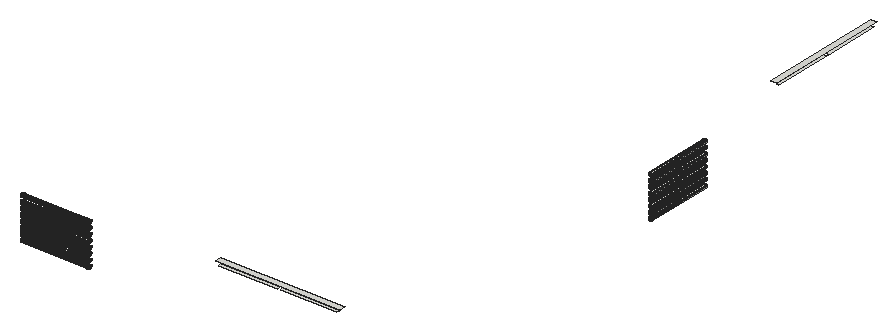
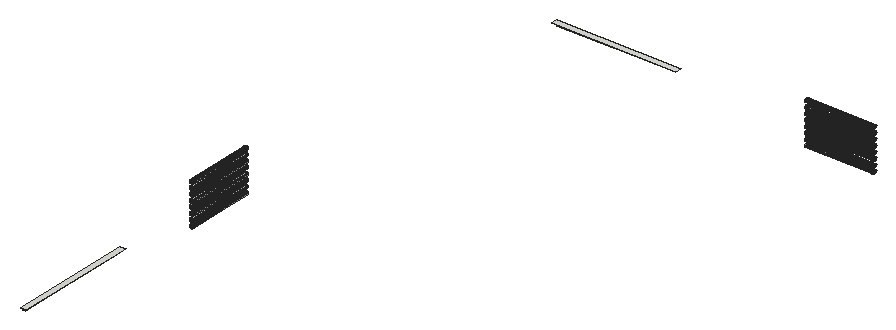
# SketchUp Ruby script. Lengths in inches.
U = 1.inch
M = Sketchup.active_model
def pt(a) = Geom::Point3d.new(a.map { |v| v * U })
def face(e, loops, mat)
  f = e.add_face(loops[0].map { |a| pt(a) })
  loops[1..].each { |l| e.add_face(l.map { |a| pt(a) }).erase! }
  f.material = f.back_material = mat if mat
  f
end
# faces: each face lists its corners as indices into pts; further lists are holes
def faces(e, pts, list, mat = nil) = list.each { |f| face(e, (f[0].is_a?(Array) ? f : [f]).map { |l| l.map { |i| pts[i] } }, mat) }
# xy, xz, yz: faces in a plane at the given z, y or x. An outline is a flat list of corners, or four numbers for a rectangle; further outlines are holes
def ring(l) = l.size == 4 ? [[l[0], l[1]], [l[2], l[1]], [l[2], l[3]], [l[0], l[3]]] : l.each_slice(2).to_a
def flat(e, list, mat, &to3) = list.each { |f| face(e, (f[0].is_a?(Array) ? f : [f]).map { |l| ring(l).map { |u, v| to3.(u, v) } }, mat) }
def xy(e, z, list, mat = nil) = flat(e, list, mat) { |x, y| [x, y, z] }
def xz(e, y, list, mat = nil) = flat(e, list, mat) { |x, z| [x, y, z] }
def yz(e, x, list, mat = nil) = flat(e, list, mat) { |y, z| [x, y, z] }
def lines(e, pts, list) = list.each { |a, b| e.add_line(pt(pts[a]), pt(pts[b])) }
# prism: a flat outline (further loops are holes) pulled along v
def prism(e, loops, v, mat = nil)
  f = face(e, loops, mat); d = Geom::Vector3d.new(v.map { |x| x * U })
  f.pushpull(f.normal.samedirection?(d) ? d.length : -d.length)
end
def box(e, o, s, mat = nil) = prism(e, [[o, [o[0] + s[0], o[1], o[2]], [o[0] + s[0], o[1] + s[1], o[2]], [o[0], o[1] + s[1], o[2]]]], [0, 0, s[2]], mat)
def at(x, y, z, deg = 0) = Geom::Transformation.translation(pt([x, y, z])) * Geom::Transformation.rotation(ORIGIN, Z_AXIS, deg.degrees)
def axes(o, x, y, z) = Geom::Transformation.new([*x, 0, *y, 0, *z, 0, *pt(o).to_a, 1])
def part(name) = M.definitions.add(name)
# library, detail: a bought-in or finely detailed component or shape, given as its bounding box
def library(name, o, s) = part(name).tap { |d| box(d.entities, o, s) }
def detail(e, o, s) = box(e.add_group.entities, o, s)
def put(e, d, t, mat = nil) = e.add_instance(d, t).tap { |i| i.material = mat if mat }
def group(e, t, mat = nil) = e.add_group.tap { |g| g.transformation = t; g.material = mat if mat }.entities
root = M.entities
xy(root,1007.61,[[1161.2,84.8125,1285.04,90.8125],[1291.04,84.8125,1408.89,90.8125],[1494,1126.01,1500,1249.86],[1494,1255.86,1500,1373.7]])
xy(root,1013.61,[[1155.2,84.8125,1414.89,96.8125],[1488,1120.01,1500,1379.7]])
p = [[922.01,48.34,933.02],[922.01,47.38,933.14],[778.64,47.38,933.14],[778.64,48.34,933.02],[922.01,49.29,933.14],[778.64,49.29,933.14],
  [1535.52,886.83,933.14],[1536.47,886.83,933.02],[1536.47,743.45,933.02],[1535.52,743.45,933.14],[1537.43,886.83,933.14],[1537.43,743.45,933.14],
  [922.01,46.5,933.51],[778.64,46.5,933.51],[922.01,50.18,933.51],[778.64,50.18,933.51],[1534.63,886.83,933.51],[1534.63,743.45,933.51],
  [1538.32,886.83,933.51],[1538.32,743.45,933.51],[922.01,45.73,934.1],[778.64,45.73,934.1],[922.01,50.95,934.1],[778.64,50.95,934.1],
  [1533.87,886.83,934.1],[1533.87,743.45,934.1],[1539.08,886.83,934.1],[1539.08,743.45,934.1],[922.01,45.15,934.86],[778.64,45.15,934.86],
  [922.01,51.53,934.86],[778.64,51.53,934.86],[1533.28,886.83,934.86],[1533.28,743.45,934.86],[1539.67,886.83,934.86],[1539.67,743.45,934.86],
  [922.01,44.78,935.75],[778.64,44.78,935.75],[922.01,51.9,935.75],[778.64,51.9,935.75],[1532.91,886.83,935.75],[1532.91,743.45,935.75],
  [1540.03,886.83,935.75],[1540.03,743.45,935.75],[922.01,44.65,936.7],[778.64,44.65,936.7],[922.01,52.03,936.7],[778.64,52.03,936.7],
  [1532.79,886.83,936.7],[1532.79,743.45,936.7],[1540.16,886.83,936.7],[1540.16,743.45,936.7],[922.01,44.78,937.66],[778.64,44.78,937.66],
  [922.01,51.9,937.66],[778.64,51.9,937.66],[1532.91,886.83,937.66],[1532.91,743.45,937.66],[1540.03,886.83,937.66],[1540.03,743.45,937.66],
  [922.01,45.15,938.55],[778.64,45.15,938.55],[922.01,51.53,938.55],[778.64,51.53,938.55],[1533.28,886.83,938.55],[1533.28,743.45,938.55],
  [1539.67,886.83,938.55],[1539.67,743.45,938.55],[922.01,45.73,939.3125],[778.64,45.73,939.3125],[922.01,50.95,939.3125],[778.64,50.95,939.3125],
  [1533.87,886.83,939.3125],[1533.87,743.45,939.3125],[1539.08,886.83,939.3125],[1539.08,743.45,939.3125],[922.01,46.5,939.9],[778.64,46.5,939.9],
  [922.01,50.18,939.9],[778.64,50.18,939.9],[1534.63,886.83,939.9],[1534.63,743.45,939.9],[1538.32,886.83,939.9],[1538.32,743.45,939.9],
  [922.01,47.38,940.27],[778.64,47.38,940.27],[922.01,49.29,940.27],[778.64,49.29,940.27],[1535.52,886.83,940.27],[1535.52,743.45,940.27],
  [1537.43,886.83,940.27],[1537.43,743.45,940.27],[922.01,48.34,940.39],[778.64,48.34,940.39],[1536.47,886.83,940.39],[1536.47,743.45,940.39],
  [922.01,48.34,945.02],[922.01,47.38,945.14],[778.64,47.38,945.14],[778.64,48.34,945.02],[922.01,49.29,945.14],[778.64,49.29,945.14],
  [1535.52,886.83,945.14],[1536.47,886.83,945.02],[1536.47,743.45,945.02],[1535.52,743.45,945.14],[1537.43,886.83,945.14],[1537.43,743.45,945.14],
  [922.01,46.5,945.51],[778.64,46.5,945.51],[922.01,50.18,945.51],[778.64,50.18,945.51],[1534.63,886.83,945.51],[1534.63,743.45,945.51],
  [1538.32,886.83,945.51],[1538.32,743.45,945.51],[922.01,45.73,946.1],[778.64,45.73,946.1],[922.01,50.95,946.1],[778.64,50.95,946.1],
  [1533.87,886.83,946.1],[1533.87,743.45,946.1],[1539.08,886.83,946.1],[1539.08,743.45,946.1],[922.01,45.15,946.86],[778.64,45.15,946.86],
  [922.01,51.53,946.86],[778.64,51.53,946.86],[1533.28,886.83,946.86],[1533.28,743.45,946.86],[1539.67,886.83,946.86],[1539.67,743.45,946.86],
  [922.01,44.78,947.75],[778.64,44.78,947.75],[922.01,51.9,947.75],[778.64,51.9,947.75],[1532.91,886.83,947.75],[1532.91,743.45,947.75],
  [1540.03,886.83,947.75],[1540.03,743.45,947.75],[922.01,44.65,948.7],[778.64,44.65,948.7],[922.01,52.03,948.7],[778.64,52.03,948.7],
  [1532.79,886.83,948.7],[1532.79,743.45,948.7],[1540.16,886.83,948.7],[1540.16,743.45,948.7],[922.01,44.78,949.66],[778.64,44.78,949.66],
  [922.01,51.9,949.66],[778.64,51.9,949.66],[1532.91,886.83,949.66],[1532.91,743.45,949.66],[1540.03,886.83,949.66],[1540.03,743.45,949.66],
  [922.01,45.15,950.55],[778.64,45.15,950.55],[922.01,51.53,950.55],[778.64,51.53,950.55],[1533.28,886.83,950.55],[1533.28,743.45,950.55],
  [1539.67,886.83,950.55],[1539.67,743.45,950.55],[922.01,45.73,951.3125],[778.64,45.73,951.3125],[922.01,50.95,951.3125],[778.64,50.95,951.3125],
  [1533.87,886.83,951.3125],[1533.87,743.45,951.3125],[1539.08,886.83,951.3125],[1539.08,743.45,951.3125],[922.01,46.5,951.9],[778.64,46.5,951.9],
  [922.01,50.18,951.9],[778.64,50.18,951.9],[1534.63,886.83,951.9],[1534.63,743.45,951.9],[1538.32,886.83,951.9],[1538.32,743.45,951.9],
  [922.01,47.38,952.27],[778.64,47.38,952.27],[922.01,49.29,952.27],[778.64,49.29,952.27],[1535.52,886.83,952.27],[1535.52,743.45,952.27],
  [1537.43,886.83,952.27],[1537.43,743.45,952.27],[922.01,48.34,952.39],[778.64,48.34,952.39],[1536.47,886.83,952.39],[1536.47,743.45,952.39],
  [922.01,48.34,957.02],[922.01,47.38,957.14],[778.64,47.38,957.14],[778.64,48.34,957.02],[922.01,49.29,957.14],[778.64,49.29,957.14],
  [1535.52,886.83,957.14],[1536.47,886.83,957.02],[1536.47,743.45,957.02],[1535.52,743.45,957.14],[1537.43,886.83,957.14],[1537.43,743.45,957.14],
  [922.01,46.5,957.51],[778.64,46.5,957.51],[922.01,50.18,957.51],[778.64,50.18,957.51],[1534.63,886.83,957.51],[1534.63,743.45,957.51],
  [1538.32,886.83,957.51],[1538.32,743.45,957.51],[922.01,45.73,958.1],[778.64,45.73,958.1],[922.01,50.95,958.1],[778.64,50.95,958.1],
  [1533.87,886.83,958.1],[1533.87,743.45,958.1],[1539.08,886.83,958.1],[1539.08,743.45,958.1],[922.01,45.15,958.86],[778.64,45.15,958.86],
  [922.01,51.53,958.86],[778.64,51.53,958.86],[1533.28,886.83,958.86],[1533.28,743.45,958.86],[1539.67,886.83,958.86],[1539.67,743.45,958.86],
  [922.01,44.78,959.75],[778.64,44.78,959.75],[922.01,51.9,959.75],[778.64,51.9,959.75],[1532.91,886.83,959.75],[1532.91,743.45,959.75],
  [1540.03,886.83,959.75],[1540.03,743.45,959.75],[922.01,44.65,960.7],[778.64,44.65,960.7],[922.01,52.03,960.7],[778.64,52.03,960.7],
  [1532.79,886.83,960.7],[1532.79,743.45,960.7],[1540.16,886.83,960.7],[1540.16,743.45,960.7],[922.01,44.78,961.66],[778.64,44.78,961.66],
  [922.01,51.9,961.66],[778.64,51.9,961.66],[1532.91,886.83,961.66],[1532.91,743.45,961.66],[1540.03,886.83,961.66],[1540.03,743.45,961.66],
  [922.01,45.15,962.55],[778.64,45.15,962.55],[922.01,51.53,962.55],[778.64,51.53,962.55],[1533.28,886.83,962.55],[1533.28,743.45,962.55],
  [1539.67,886.83,962.55],[1539.67,743.45,962.55],[922.01,45.73,963.3125],[778.64,45.73,963.3125],[922.01,50.95,963.3125],[778.64,50.95,963.3125],
  [1533.87,886.83,963.3125],[1533.87,743.45,963.3125],[1539.08,886.83,963.3125],[1539.08,743.45,963.3125],[922.01,46.5,963.9],[778.64,46.5,963.9],
  [922.01,50.18,963.9],[778.64,50.18,963.9],[1534.63,886.83,963.9],[1534.63,743.45,963.9],[1538.32,886.83,963.9],[1538.32,743.45,963.9],
  [922.01,47.38,964.27],[778.64,47.38,964.27],[922.01,49.29,964.27],[778.64,49.29,964.27],[1535.52,886.83,964.27],[1535.52,743.45,964.27],
  [1537.43,886.83,964.27],[1537.43,743.45,964.27],[922.01,48.34,964.39],[778.64,48.34,964.39],[1536.47,886.83,964.39],[1536.47,743.45,964.39],
  [922.01,48.34,969.02],[922.01,47.38,969.14],[778.64,47.38,969.14],[778.64,48.34,969.02],[922.01,49.29,969.14],[778.64,49.29,969.14],
  [1535.52,886.83,969.14],[1536.47,886.83,969.02],[1536.47,743.45,969.02],[1535.52,743.45,969.14],[1537.43,886.83,969.14],[1537.43,743.45,969.14],
  [922.01,46.5,969.51],[778.64,46.5,969.51],[922.01,50.18,969.51],[778.64,50.18,969.51],[1534.63,886.83,969.51],[1534.63,743.45,969.51],
  [1538.32,886.83,969.51],[1538.32,743.45,969.51],[922.01,45.73,970.1],[778.64,45.73,970.1],[922.01,50.95,970.1],[778.64,50.95,970.1],
  [1533.87,886.83,970.1],[1533.87,743.45,970.1],[1539.08,886.83,970.1],[1539.08,743.45,970.1],[922.01,45.15,970.86],[778.64,45.15,970.86],
  [922.01,51.53,970.86],[778.64,51.53,970.86],[1533.28,886.83,970.86],[1533.28,743.45,970.86],[1539.67,886.83,970.86],[1539.67,743.45,970.86],
  [922.01,44.78,971.75],[778.64,44.78,971.75],[922.01,51.9,971.75],[778.64,51.9,971.75],[1532.91,886.83,971.75],[1532.91,743.45,971.75],
  [1540.03,886.83,971.75],[1540.03,743.45,971.75],[922.01,44.65,972.7],[778.64,44.65,972.7],[922.01,52.03,972.7],[778.64,52.03,972.7],
  [1532.79,886.83,972.7],[1532.79,743.45,972.7],[1540.16,886.83,972.7],[1540.16,743.45,972.7],[922.01,44.78,973.66],[778.64,44.78,973.66],
  [922.01,51.9,973.66],[778.64,51.9,973.66],[1532.91,886.83,973.66],[1532.91,743.45,973.66],[1540.03,886.83,973.66],[1540.03,743.45,973.66],
  [922.01,45.15,974.55],[778.64,45.15,974.55],[922.01,51.53,974.55],[778.64,51.53,974.55],[1533.28,886.83,974.55],[1533.28,743.45,974.55],
  [1539.67,886.83,974.55],[1539.67,743.45,974.55],[922.01,45.73,975.3125],[778.64,45.73,975.3125],[922.01,50.95,975.3125],[778.64,50.95,975.3125],
  [1533.87,886.83,975.3125],[1533.87,743.45,975.3125],[1539.08,886.83,975.3125],[1539.08,743.45,975.3125],[922.01,46.5,975.9],[778.64,46.5,975.9],
  [922.01,50.18,975.9],[778.64,50.18,975.9],[1534.63,886.83,975.9],[1534.63,743.45,975.9],[1538.32,886.83,975.9],[1538.32,743.45,975.9],
  [922.01,47.38,976.27],[778.64,47.38,976.27],[922.01,49.29,976.27],[778.64,49.29,976.27],[1535.52,886.83,976.27],[1535.52,743.45,976.27],
  [1537.43,886.83,976.27],[1537.43,743.45,976.27],[922.01,48.34,976.39],[778.64,48.34,976.39],[1536.47,886.83,976.39],[1536.47,743.45,976.39],
  [922.01,48.34,981.02],[922.01,47.38,981.14],[778.64,47.38,981.14],[778.64,48.34,981.02],[922.01,49.29,981.14],[778.64,49.29,981.14],
  [1535.52,886.83,981.14],[1536.47,886.83,981.02],[1536.47,743.45,981.02],[1535.52,743.45,981.14],[1537.43,886.83,981.14],[1537.43,743.45,981.14],
  [922.01,46.5,981.51],[778.64,46.5,981.51],[922.01,50.18,981.51],[778.64,50.18,981.51],[1534.63,886.83,981.51],[1534.63,743.45,981.51],
  [1538.32,886.83,981.51],[1538.32,743.45,981.51],[922.01,45.73,982.1],[778.64,45.73,982.1],[922.01,50.95,982.1],[778.64,50.95,982.1],
  [1533.87,886.83,982.1],[1533.87,743.45,982.1],[1539.08,886.83,982.1],[1539.08,743.45,982.1],[922.01,45.15,982.86],[778.64,45.15,982.86],
  [922.01,51.53,982.86],[778.64,51.53,982.86],[1533.28,886.83,982.86],[1533.28,743.45,982.86],[1539.67,886.83,982.86],[1539.67,743.45,982.86],
  [922.01,44.78,983.75],[778.64,44.78,983.75],[922.01,51.9,983.75],[778.64,51.9,983.75],[1532.91,886.83,983.75],[1532.91,743.45,983.75],
  [1540.03,886.83,983.75],[1540.03,743.45,983.75],[922.01,44.65,984.7],[778.64,44.65,984.7],[922.01,52.03,984.7],[778.64,52.03,984.7],
  [1532.79,886.83,984.7],[1532.79,743.45,984.7],[1540.16,886.83,984.7],[1540.16,743.45,984.7],[922.01,44.78,985.66],[778.64,44.78,985.66],
  [922.01,51.9,985.66],[778.64,51.9,985.66],[1532.91,886.83,985.66],[1532.91,743.45,985.66],[1540.03,886.83,985.66],[1540.03,743.45,985.66],
  [922.01,45.15,986.55],[778.64,45.15,986.55],[922.01,51.53,986.55],[778.64,51.53,986.55],[1533.28,886.83,986.55],[1533.28,743.45,986.55],
  [1539.67,886.83,986.55],[1539.67,743.45,986.55],[922.01,45.73,987.3125],[778.64,45.73,987.3125],[922.01,50.95,987.3125],[778.64,50.95,987.3125],
  [1533.87,886.83,987.3125],[1533.87,743.45,987.3125],[1539.08,886.83,987.3125],[1539.08,743.45,987.3125],[922.01,46.5,987.9],[778.64,46.5,987.9],
  [922.01,50.18,987.9],[778.64,50.18,987.9],[1534.63,886.83,987.9],[1534.63,743.45,987.9],[1538.32,886.83,987.9],[1538.32,743.45,987.9],
  [922.01,47.38,988.27],[778.64,47.38,988.27],[922.01,49.29,988.27],[778.64,49.29,988.27],[1535.52,886.83,988.27],[1535.52,743.45,988.27],
  [1537.43,886.83,988.27],[1537.43,743.45,988.27],[922.01,48.34,988.39],[778.64,48.34,988.39],[1536.47,886.83,988.39],[1536.47,743.45,988.39],
  [922.01,48.34,993.02],[922.01,47.38,993.14],[778.64,47.38,993.14],[778.64,48.34,993.02],[922.01,49.29,993.14],[778.64,49.29,993.14],
  [1535.52,886.83,993.14],[1536.47,886.83,993.02],[1536.47,743.45,993.02],[1535.52,743.45,993.14],[1537.43,886.83,993.14],[1537.43,743.45,993.14],
  [922.01,46.5,993.51],[778.64,46.5,993.51],[922.01,50.18,993.51],[778.64,50.18,993.51],[1534.63,886.83,993.51],[1534.63,743.45,993.51],
  [1538.32,886.83,993.51],[1538.32,743.45,993.51],[922.01,45.73,994.1],[778.64,45.73,994.1],[922.01,50.95,994.1],[778.64,50.95,994.1],
  [1533.87,886.83,994.1],[1533.87,743.45,994.1],[1539.08,886.83,994.1],[1539.08,743.45,994.1],[922.01,45.15,994.86],[778.64,45.15,994.86],
  [922.01,51.53,994.86],[778.64,51.53,994.86],[1533.28,886.83,994.86],[1533.28,743.45,994.86],[1539.67,886.83,994.86],[1539.67,743.45,994.86],
  [922.01,44.78,995.75],[778.64,44.78,995.75],[922.01,51.9,995.75],[778.64,51.9,995.75],[1532.91,886.83,995.75],[1532.91,743.45,995.75],
  [1540.03,886.83,995.75],[1540.03,743.45,995.75],[922.01,44.65,996.7],[778.64,44.65,996.7],[922.01,52.03,996.7],[778.64,52.03,996.7],
  [1532.79,886.83,996.7],[1532.79,743.45,996.7],[1540.16,886.83,996.7],[1540.16,743.45,996.7],[922.01,44.78,997.66],[778.64,44.78,997.66],
  [922.01,51.9,997.66],[778.64,51.9,997.66],[1532.91,886.83,997.66],[1532.91,743.45,997.66],[1540.03,886.83,997.66],[1540.03,743.45,997.66],
  [922.01,45.15,998.55],[778.64,45.15,998.55],[922.01,51.53,998.55],[778.64,51.53,998.55],[1533.28,886.83,998.55],[1533.28,743.45,998.55],
  [1539.67,886.83,998.55],[1539.67,743.45,998.55],[922.01,45.73,999.3125],[778.64,45.73,999.3125],[922.01,50.95,999.3125],[778.64,50.95,999.3125],
  [1533.87,886.83,999.3125],[1533.87,743.45,999.3125],[1539.08,886.83,999.3125],[1539.08,743.45,999.3125],[922.01,46.5,999.9],[778.64,46.5,999.9],
  [922.01,50.18,999.9],[778.64,50.18,999.9],[1534.63,886.83,999.9],[1534.63,743.45,999.9],[1538.32,886.83,999.9],[1538.32,743.45,999.9],
  [922.01,47.38,1000.27],[778.64,47.38,1000.27],[922.01,49.29,1000.27],[778.64,49.29,1000.27],[1535.52,886.83,1000.27],[1535.52,743.45,1000.27],
  [1537.43,886.83,1000.27],[1537.43,743.45,1000.27],[922.01,48.34,1000.39],[778.64,48.34,1000.39],[1536.47,886.83,1000.39],[1536.47,743.45,1000.39],
  [922.01,48.34,1005.02],[922.01,47.38,1005.14],[778.64,47.38,1005.14],[778.64,48.34,1005.02],[922.01,49.29,1005.14],[778.64,49.29,1005.14],
  [1535.52,886.83,1005.14],[1536.47,886.83,1005.02],[1536.47,743.45,1005.02],[1535.52,743.45,1005.14],[1537.43,886.83,1005.14],[1537.43,743.45,1005.14],
  [922.01,46.5,1005.51],[778.64,46.5,1005.51],[922.01,50.18,1005.51],[778.64,50.18,1005.51],[1534.63,886.83,1005.51],[1534.63,743.45,1005.51],
  [1538.32,886.83,1005.51],[1538.32,743.45,1005.51],[922.01,45.73,1006.1],[778.64,45.73,1006.1],[922.01,50.95,1006.1],[778.64,50.95,1006.1],
  [1533.87,886.83,1006.1],[1533.87,743.45,1006.1],[1539.08,886.83,1006.1],[1539.08,743.45,1006.1],[922.01,45.15,1006.86],[778.64,45.15,1006.86],
  [922.01,51.53,1006.86],[778.64,51.53,1006.86],[1533.28,886.83,1006.86],[1533.28,743.45,1006.86],[1539.67,886.83,1006.86],[1539.67,743.45,1006.86],
  [922.01,44.78,1007.75],[778.64,44.78,1007.75],[922.01,51.9,1007.75],[778.64,51.9,1007.75],[1532.91,886.83,1007.75],[1532.91,743.45,1007.75],
  [1540.03,886.83,1007.75],[1540.03,743.45,1007.75],[922.01,44.65,1008.7],[778.64,44.65,1008.7],[922.01,52.03,1008.7],[778.64,52.03,1008.7],
  [1532.79,886.83,1008.7],[1532.79,743.45,1008.7],[1540.16,886.83,1008.7],[1540.16,743.45,1008.7],[922.01,44.78,1009.66],[778.64,44.78,1009.66],
  [922.01,51.9,1009.66],[778.64,51.9,1009.66],[1532.91,886.83,1009.66],[1532.91,743.45,1009.66],[1540.03,886.83,1009.66],[1540.03,743.45,1009.66],
  [922.01,45.15,1010.55],[778.64,45.15,1010.55],[922.01,51.53,1010.55],[778.64,51.53,1010.55],[1533.28,886.83,1010.55],[1533.28,743.45,1010.55],
  [1539.67,886.83,1010.55],[1539.67,743.45,1010.55],[922.01,45.73,1011.3125],[778.64,45.73,1011.3125],[922.01,50.95,1011.3125],[778.64,50.95,1011.3125],
  [1533.87,886.83,1011.3125],[1533.87,743.45,1011.3125],[1539.08,886.83,1011.3125],[1539.08,743.45,1011.3125],[922.01,46.5,1011.9],[778.64,46.5,1011.9],
  [922.01,50.18,1011.9],[778.64,50.18,1011.9],[1534.63,886.83,1011.9],[1534.63,743.45,1011.9],[1538.32,886.83,1011.9],[1538.32,743.45,1011.9],
  [922.01,47.38,1012.27],[778.64,47.38,1012.27],[922.01,49.29,1012.27],[778.64,49.29,1012.27],[1535.52,886.83,1012.27],[1535.52,743.45,1012.27],
  [1537.43,886.83,1012.27],[1537.43,743.45,1012.27],[922.01,48.34,1012.39],[778.64,48.34,1012.39],[1536.47,886.83,1012.39],[1536.47,743.45,1012.39],
  [922.01,48.34,1017.02],[922.01,47.38,1017.14],[778.64,47.38,1017.14],[778.64,48.34,1017.02],[922.01,49.29,1017.14],[778.64,49.29,1017.14],
  [1535.52,886.83,1017.14],[1536.47,886.83,1017.02],[1536.47,743.45,1017.02],[1535.52,743.45,1017.14],[1537.43,886.83,1017.14],[1537.43,743.45,1017.14],
  [922.01,46.5,1017.51],[778.64,46.5,1017.51],[922.01,50.18,1017.51],[778.64,50.18,1017.51],[1534.63,886.83,1017.51],[1534.63,743.45,1017.51],
  [1538.32,886.83,1017.51],[1538.32,743.45,1017.51],[922.01,45.73,1018.1],[778.64,45.73,1018.1],[922.01,50.95,1018.1],[778.64,50.95,1018.1],
  [1533.87,886.83,1018.1],[1533.87,743.45,1018.1],[1539.08,886.83,1018.1],[1539.08,743.45,1018.1],[922.01,45.15,1018.86],[778.64,45.15,1018.86],
  [922.01,51.53,1018.86],[778.64,51.53,1018.86],[1533.28,886.83,1018.86],[1533.28,743.45,1018.86],[1539.67,886.83,1018.86],[1539.67,743.45,1018.86],
  [922.01,44.78,1019.75],[778.64,44.78,1019.75],[922.01,51.9,1019.75],[778.64,51.9,1019.75],[1532.91,886.83,1019.75],[1532.91,743.45,1019.75],
  [1540.03,886.83,1019.75],[1540.03,743.45,1019.75],[922.01,44.65,1020.7],[778.64,44.65,1020.7],[922.01,52.03,1020.7],[778.64,52.03,1020.7],
  [1532.79,886.83,1020.7],[1532.79,743.45,1020.7],[1540.16,886.83,1020.7],[1540.16,743.45,1020.7],[922.01,44.78,1021.66],[778.64,44.78,1021.66],
  [922.01,51.9,1021.66],[778.64,51.9,1021.66],[1532.91,886.83,1021.66],[1532.91,743.45,1021.66],[1540.03,886.83,1021.66],[1540.03,743.45,1021.66],
  [922.01,45.15,1022.55],[778.64,45.15,1022.55],[922.01,51.53,1022.55],[778.64,51.53,1022.55],[1533.28,886.83,1022.55],[1533.28,743.45,1022.55],
  [1539.67,886.83,1022.55],[1539.67,743.45,1022.55],[922.01,45.73,1023.3125],[778.64,45.73,1023.3125],[922.01,50.95,1023.3125],[778.64,50.95,1023.3125],
  [1533.87,886.83,1023.3125],[1533.87,743.45,1023.3125],[1539.08,886.83,1023.3125],[1539.08,743.45,1023.3125],[922.01,46.5,1023.9],[778.64,46.5,1023.9],
  [922.01,50.18,1023.9],[778.64,50.18,1023.9],[1534.63,886.83,1023.9],[1534.63,743.45,1023.9],[1538.32,886.83,1023.9],[1538.32,743.45,1023.9],
  [922.01,47.38,1024.27],[778.64,47.38,1024.27],[922.01,49.29,1024.27],[778.64,49.29,1024.27],[1535.52,886.83,1024.27],[1535.52,743.45,1024.27],
  [1537.43,886.83,1024.27],[1537.43,743.45,1024.27],[922.01,48.34,1024.39],[778.64,48.34,1024.39],[1536.47,886.83,1024.39],[1536.47,743.45,1024.39]]
faces(root,p,[[0,1,2,3],[4,0,3,5],[6,7,8,9],[7,10,11,8],[1,12,13,2],[14,4,5,15],[16,6,9,17],[10,18,19,11],
  [12,20,21,13],[22,14,15,23],[24,16,17,25],[18,26,27,19],[20,28,29,21],[30,22,23,31],[32,24,25,33],[26,34,35,27],
  [28,36,37,29],[38,30,31,39],[40,32,33,41],[34,42,43,35],[36,44,45,37],[46,38,39,47],[48,40,41,49],[42,50,51,43],
  [44,52,53,45],[54,46,47,55],[56,48,49,57],[50,58,59,51],[52,60,61,53],[62,54,55,63],[64,56,57,65],[58,66,67,59],
  [60,68,69,61],[70,62,63,71],[72,64,65,73],[66,74,75,67],[68,76,77,69],[78,70,71,79],[80,72,73,81],[74,82,83,75],
  [76,84,85,77],[86,78,79,87],[88,80,81,89],[82,90,91,83],[84,92,93,85],[92,86,87,93],[94,88,89,95],[90,94,95,91],
  [96,97,98,99],[100,96,99,101],[102,103,104,105],[103,106,107,104],[97,108,109,98],[110,100,101,111],[112,102,105,113],[106,114,115,107],
  [108,116,117,109],[118,110,111,119],[120,112,113,121],[114,122,123,115],[116,124,125,117],[126,118,119,127],[128,120,121,129],[122,130,131,123],
  [124,132,133,125],[134,126,127,135],[136,128,129,137],[130,138,139,131],[132,140,141,133],[142,134,135,143],[144,136,137,145],[138,146,147,139],
  [140,148,149,141],[150,142,143,151],[152,144,145,153],[146,154,155,147],[148,156,157,149],[158,150,151,159],[160,152,153,161],[154,162,163,155],
  [156,164,165,157],[166,158,159,167],[168,160,161,169],[162,170,171,163],[164,172,173,165],[174,166,167,175],[176,168,169,177],[170,178,179,171],
  [172,180,181,173],[182,174,175,183],[184,176,177,185],[178,186,187,179],[180,188,189,181],[188,182,183,189],[190,184,185,191],[186,190,191,187],
  [192,193,194,195],[196,192,195,197],[198,199,200,201],[199,202,203,200],[193,204,205,194],[206,196,197,207],[208,198,201,209],[202,210,211,203],
  [204,212,213,205],[214,206,207,215],[216,208,209,217],[210,218,219,211],[212,220,221,213],[222,214,215,223],[224,216,217,225],[218,226,227,219],
  [220,228,229,221],[230,222,223,231],[232,224,225,233],[226,234,235,227],[228,236,237,229],[238,230,231,239],[240,232,233,241],[234,242,243,235],
  [236,244,245,237],[246,238,239,247],[248,240,241,249],[242,250,251,243],[244,252,253,245],[254,246,247,255],[256,248,249,257],[250,258,259,251],
  [252,260,261,253],[262,254,255,263],[264,256,257,265],[258,266,267,259],[260,268,269,261],[270,262,263,271],[272,264,265,273],[266,274,275,267],
  [268,276,277,269],[278,270,271,279],[280,272,273,281],[274,282,283,275],[276,284,285,277],[284,278,279,285],[286,280,281,287],[282,286,287,283],
  [288,289,290,291],[292,288,291,293],[294,295,296,297],[295,298,299,296],[289,300,301,290],[302,292,293,303],[304,294,297,305],[298,306,307,299],
  [300,308,309,301],[310,302,303,311],[312,304,305,313],[306,314,315,307],[308,316,317,309],[318,310,311,319],[320,312,313,321],[314,322,323,315],
  [316,324,325,317],[326,318,319,327],[328,320,321,329],[322,330,331,323],[324,332,333,325],[334,326,327,335],[336,328,329,337],[330,338,339,331],
  [332,340,341,333],[342,334,335,343],[344,336,337,345],[338,346,347,339],[340,348,349,341],[350,342,343,351],[352,344,345,353],[346,354,355,347],
  [348,356,357,349],[358,350,351,359],[360,352,353,361],[354,362,363,355],[356,364,365,357],[366,358,359,367],[368,360,361,369],[362,370,371,363],
  [364,372,373,365],[374,366,367,375],[376,368,369,377],[370,378,379,371],[372,380,381,373],[380,374,375,381],[382,376,377,383],[378,382,383,379],
  [384,385,386,387],[388,384,387,389],[390,391,392,393],[391,394,395,392],[385,396,397,386],[398,388,389,399],[400,390,393,401],[394,402,403,395],
  [396,404,405,397],[406,398,399,407],[408,400,401,409],[402,410,411,403],[404,412,413,405],[414,406,407,415],[416,408,409,417],[410,418,419,411],
  [412,420,421,413],[422,414,415,423],[424,416,417,425],[418,426,427,419],[420,428,429,421],[430,422,423,431],[432,424,425,433],[426,434,435,427],
  [428,436,437,429],[438,430,431,439],[440,432,433,441],[434,442,443,435],[436,444,445,437],[446,438,439,447],[448,440,441,449],[442,450,451,443],
  [444,452,453,445],[454,446,447,455],[456,448,449,457],[450,458,459,451],[452,460,461,453],[462,454,455,463],[464,456,457,465],[458,466,467,459],
  [460,468,469,461],[470,462,463,471],[472,464,465,473],[466,474,475,467],[468,476,477,469],[476,470,471,477],[478,472,473,479],[474,478,479,475],
  [480,481,482,483],[484,480,483,485],[486,487,488,489],[487,490,491,488],[481,492,493,482],[494,484,485,495],[496,486,489,497],[490,498,499,491],
  [492,500,501,493],[502,494,495,503],[504,496,497,505],[498,506,507,499],[500,508,509,501],[510,502,503,511],[512,504,505,513],[506,514,515,507],
  [508,516,517,509],[518,510,511,519],[520,512,513,521],[514,522,523,515],[516,524,525,517],[526,518,519,527],[528,520,521,529],[522,530,531,523],
  [524,532,533,525],[534,526,527,535],[536,528,529,537],[530,538,539,531],[532,540,541,533],[542,534,535,543],[544,536,537,545],[538,546,547,539],
  [540,548,549,541],[550,542,543,551],[552,544,545,553],[546,554,555,547],[548,556,557,549],[558,550,551,559],[560,552,553,561],[554,562,563,555],
  [556,564,565,557],[566,558,559,567],[568,560,561,569],[562,570,571,563],[564,572,573,565],[572,566,567,573],[574,568,569,575],[570,574,575,571],
  [576,577,578,579],[580,576,579,581],[582,583,584,585],[583,586,587,584],[577,588,589,578],[590,580,581,591],[592,582,585,593],[586,594,595,587],
  [588,596,597,589],[598,590,591,599],[600,592,593,601],[594,602,603,595],[596,604,605,597],[606,598,599,607],[608,600,601,609],[602,610,611,603],
  [604,612,613,605],[614,606,607,615],[616,608,609,617],[610,618,619,611],[612,620,621,613],[622,614,615,623],[624,616,617,625],[618,626,627,619],
  [620,628,629,621],[630,622,623,631],[632,624,625,633],[626,634,635,627],[628,636,637,629],[638,630,631,639],[640,632,633,641],[634,642,643,635],
  [636,644,645,637],[646,638,639,647],[648,640,641,649],[642,650,651,643],[644,652,653,645],[654,646,647,655],[656,648,649,657],[650,658,659,651],
  [652,660,661,653],[662,654,655,663],[664,656,657,665],[658,666,667,659],[660,668,669,661],[668,662,663,669],[670,664,665,671],[666,670,671,667],
  [672,673,674,675],[676,672,675,677],[678,679,680,681],[679,682,683,680],[673,684,685,674],[686,676,677,687],[688,678,681,689],[682,690,691,683],
  [684,692,693,685],[694,686,687,695],[696,688,689,697],[690,698,699,691],[692,700,701,693],[702,694,695,703],[704,696,697,705],[698,706,707,699],
  [700,708,709,701],[710,702,703,711],[712,704,705,713],[706,714,715,707],[708,716,717,709],[718,710,711,719],[720,712,713,721],[714,722,723,715],
  [716,724,725,717],[726,718,719,727],[728,720,721,729],[722,730,731,723],[724,732,733,725],[734,726,727,735],[736,728,729,737],[730,738,739,731],
  [732,740,741,733],[742,734,735,743],[744,736,737,745],[738,746,747,739],[740,748,749,741],[750,742,743,751],[752,744,745,753],[746,754,755,747],
  [748,756,757,749],[758,750,751,759],[760,752,753,761],[754,762,763,755],[756,764,765,757],[764,758,759,765],[766,760,761,767],[762,766,767,763]])
